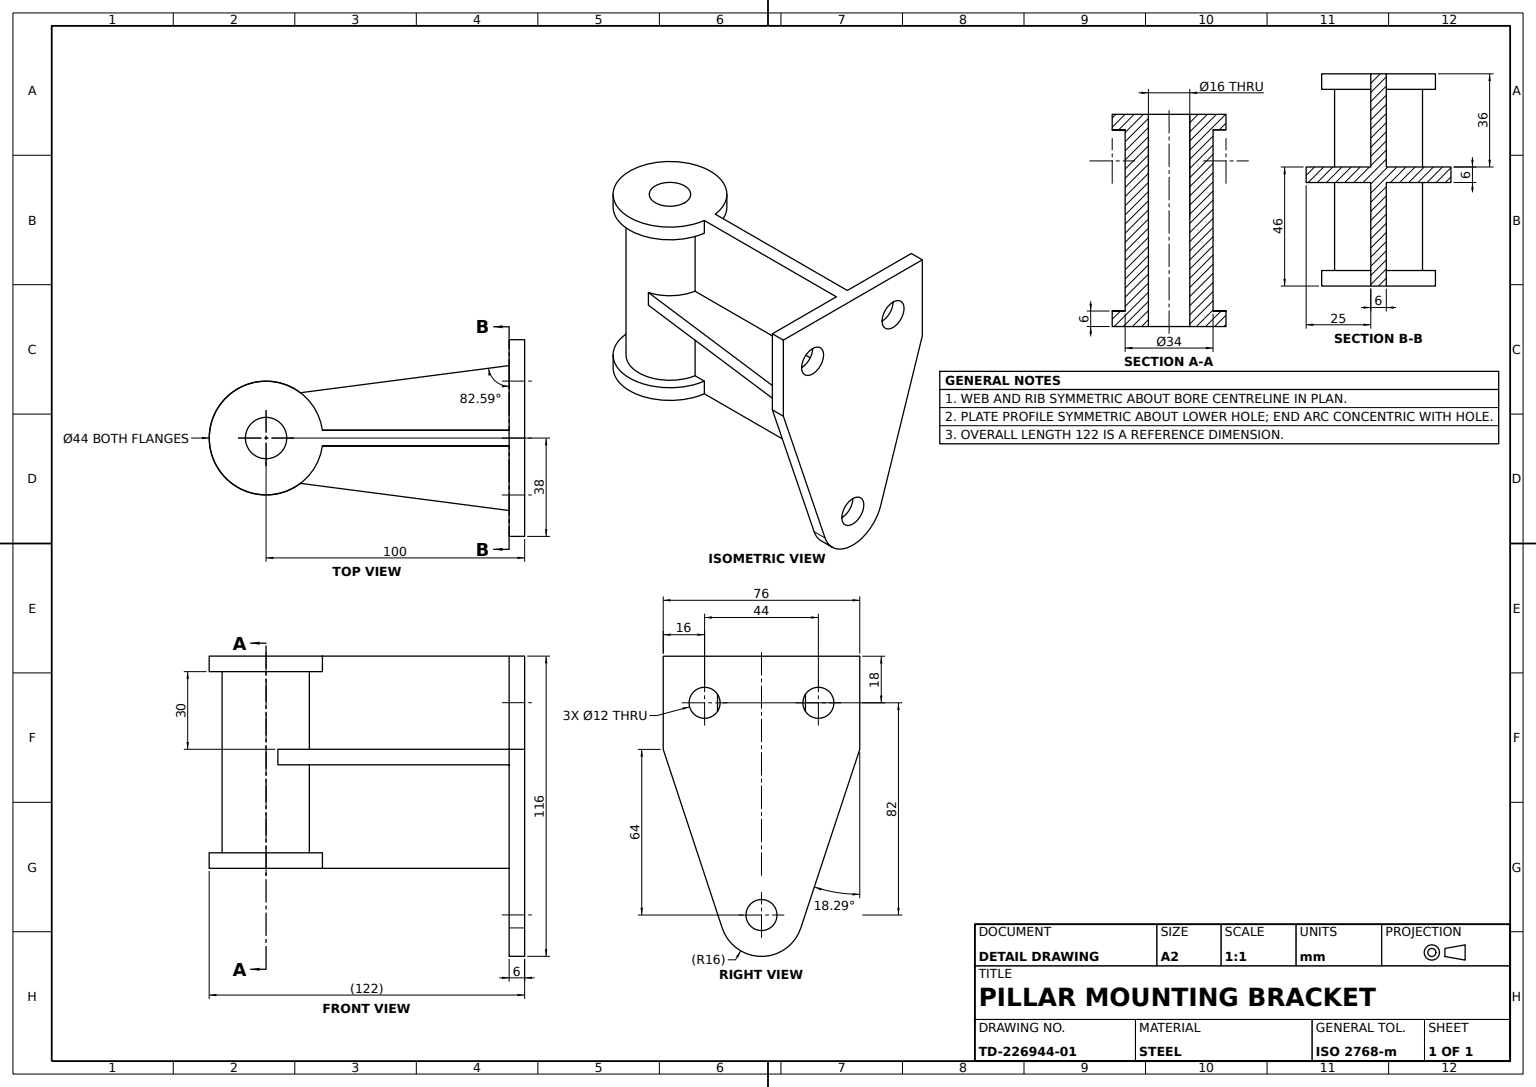
ISO-10303-21;
HEADER;
FILE_DESCRIPTION((''),'2;1');
FILE_NAME('','',(''),(''),'','','');
FILE_SCHEMA(('AUTOMOTIVE_DESIGN'));
ENDSEC;
DATA;
#1=APPLICATION_CONTEXT('');
#2=PRODUCT_CONTEXT('',#1,'mechanical');
#3=PRODUCT('','','',(#2));
#4=PRODUCT_DEFINITION_FORMATION('','',#3);
#5=PRODUCT_DEFINITION_CONTEXT('',#1,'design');
#6=PRODUCT_DEFINITION('','',#4,#5);
#7=PRODUCT_DEFINITION_SHAPE('','',#6);
#8=(LENGTH_UNIT()NAMED_UNIT(*)SI_UNIT(.MILLI.,.METRE.));
#9=(NAMED_UNIT(*)PLANE_ANGLE_UNIT()SI_UNIT($,.RADIAN.));
#10=(NAMED_UNIT(*)SI_UNIT($,.STERADIAN.)SOLID_ANGLE_UNIT());
#11=UNCERTAINTY_MEASURE_WITH_UNIT(LENGTH_MEASURE(0.005),#8,'distance_accuracy_value','');
#12=(GEOMETRIC_REPRESENTATION_CONTEXT(3)GLOBAL_UNCERTAINTY_ASSIGNED_CONTEXT((#11))GLOBAL_UNIT_ASSIGNED_CONTEXT((#8,#9,#10))REPRESENTATION_CONTEXT('',''));
#13=CARTESIAN_POINT('',(83.266799,-3.,-6.));
#14=VERTEX_POINT('',#13);
#15=CARTESIAN_POINT('',(6.,-3.,-6.));
#16=VERTEX_POINT('',#15);
#17=CARTESIAN_POINT('',(106.,-3.,-6.));
#18=DIRECTION('',(-1.,0.,0.));
#19=VECTOR('',#18,1000.);
#20=LINE('',#17,#19);
#21=EDGE_CURVE('',#14,#16,#20,.T.);
#22=ORIENTED_EDGE('',*,*,#21,.T.);
#23=CARTESIAN_POINT('',(6.,-3.,-46.));
#24=VERTEX_POINT('',#23);
#25=CARTESIAN_POINT('',(6.,-3.,36.));
#26=DIRECTION('',(0.,0.,-1.));
#27=VECTOR('',#26,1000.);
#28=LINE('',#25,#27);
#29=EDGE_CURVE('',#16,#24,#28,.T.);
#30=ORIENTED_EDGE('',*,*,#29,.T.);
#31=CARTESIAN_POINT('',(78.205505,-3.,-46.));
#32=VERTEX_POINT('',#31);
#33=DIRECTION('',(1.,0.,0.));
#34=VECTOR('',#33,1000.);
#35=LINE('',#23,#34);
#36=EDGE_CURVE('',#24,#32,#35,.T.);
#37=ORIENTED_EDGE('',*,*,#36,.T.);
#38=CARTESIAN_POINT('',(78.205505,-3.,-40.));
#39=VERTEX_POINT('',#38);
#40=LINE('',#38,#27);
#41=EDGE_CURVE('',#39,#32,#40,.T.);
#42=ORIENTED_EDGE('',*,*,#41,.F.);
#43=CARTESIAN_POINT('',(83.266799,-3.,-40.));
#44=VERTEX_POINT('',#43);
#45=CARTESIAN_POINT('',(0.,-3.,-40.));
#46=LINE('',#45,#19);
#47=EDGE_CURVE('',#39,#44,#46,.F.);
#48=ORIENTED_EDGE('',*,*,#47,.T.);
#49=CARTESIAN_POINT('',(83.266799,-3.,36.));
#50=LINE('',#49,#27);
#51=EDGE_CURVE('',#44,#14,#50,.F.);
#52=ORIENTED_EDGE('',*,*,#51,.T.);
#53=EDGE_LOOP('',(#22,#30,#37,#42,#48,#52));
#54=FACE_BOUND('',#53,.T.);
#55=CARTESIAN_POINT('',(0.,-3.,0.));
#56=DIRECTION('',(0.,-1.,0.));
#57=AXIS2_PLACEMENT_3D('',#55,#56,#26);
#58=PLANE('',#57);
#59=ADVANCED_FACE('',(#54),#58,.T.);
#60=CARTESIAN_POINT('',(83.266799,-3.,0.));
#61=VERTEX_POINT('',#60);
#62=CARTESIAN_POINT('',(83.266799,-3.,30.));
#63=VERTEX_POINT('',#62);
#64=EDGE_CURVE('',#61,#63,#50,.F.);
#65=ORIENTED_EDGE('',*,*,#64,.T.);
#66=CARTESIAN_POINT('',(78.205505,-3.,30.));
#67=VERTEX_POINT('',#66);
#68=CARTESIAN_POINT('',(0.,-3.,30.));
#69=LINE('',#68,#19);
#70=EDGE_CURVE('',#67,#63,#69,.F.);
#71=ORIENTED_EDGE('',*,*,#70,.F.);
#72=CARTESIAN_POINT('',(78.205505,-3.,36.));
#73=VERTEX_POINT('',#72);
#74=LINE('',#72,#27);
#75=EDGE_CURVE('',#73,#67,#74,.T.);
#76=ORIENTED_EDGE('',*,*,#75,.F.);
#77=VERTEX_POINT('',#25);
#78=CARTESIAN_POINT('',(106.,-3.,36.));
#79=LINE('',#78,#19);
#80=EDGE_CURVE('',#73,#77,#79,.T.);
#81=ORIENTED_EDGE('',*,*,#80,.T.);
#82=CARTESIAN_POINT('',(6.,-3.,0.));
#83=VERTEX_POINT('',#82);
#84=EDGE_CURVE('',#77,#83,#28,.T.);
#85=ORIENTED_EDGE('',*,*,#84,.T.);
#86=CARTESIAN_POINT('',(106.,-3.,0.));
#87=LINE('',#86,#19);
#88=EDGE_CURVE('',#61,#83,#87,.T.);
#89=ORIENTED_EDGE('',*,*,#88,.F.);
#90=EDGE_LOOP('',(#65,#71,#76,#81,#85,#89));
#91=FACE_BOUND('',#90,.T.);
#92=ADVANCED_FACE('',(#91),#58,.T.);
#93=CARTESIAN_POINT('',(108.,0.,-46.));
#94=VERTEX_POINT('',#93);
#95=CARTESIAN_POINT('',(100.,0.,-46.));
#96=DIRECTION('',(0.,0.,1.));
#97=AXIS2_PLACEMENT_3D('',#95,#96,#33);
#98=CIRCLE('',#97,8.);
#99=EDGE_CURVE('',#94,#94,#98,.T.);
#100=ORIENTED_EDGE('',*,*,#99,.T.);
#101=EDGE_LOOP('',(#100));
#102=FACE_BOUND('',#101,.T.);
#103=CARTESIAN_POINT('',(6.,3.,-46.));
#104=VERTEX_POINT('',#103);
#105=DIRECTION('',(0.,1.,0.));
#106=VECTOR('',#105,1000.);
#107=LINE('',#23,#106);
#108=EDGE_CURVE('',#24,#104,#107,.T.);
#109=ORIENTED_EDGE('',*,*,#108,.T.);
#110=CARTESIAN_POINT('',(78.205505,3.,-46.));
#111=VERTEX_POINT('',#110);
#112=LINE('',#103,#34);
#113=EDGE_CURVE('',#104,#111,#112,.T.);
#114=ORIENTED_EDGE('',*,*,#113,.T.);
#115=CIRCLE('',#97,22.);
#116=EDGE_CURVE('',#111,#32,#115,.F.);
#117=ORIENTED_EDGE('',*,*,#116,.T.);
#118=ORIENTED_EDGE('',*,*,#36,.F.);
#119=EDGE_LOOP('',(#109,#114,#117,#118));
#120=FACE_BOUND('',#119,.T.);
#121=AXIS2_PLACEMENT_3D('',#23,#96,#33);
#122=PLANE('',#121);
#123=ADVANCED_FACE('',(#102,#120),#122,.F.);
#124=CARTESIAN_POINT('',(83.266799,3.,-6.));
#125=VERTEX_POINT('',#124);
#126=CARTESIAN_POINT('',(6.,3.,-6.));
#127=VERTEX_POINT('',#126);
#128=CARTESIAN_POINT('',(106.,3.,-6.));
#129=LINE('',#128,#19);
#130=EDGE_CURVE('',#125,#127,#129,.T.);
#131=ORIENTED_EDGE('',*,*,#130,.F.);
#132=CARTESIAN_POINT('',(83.266799,3.,-40.));
#133=VERTEX_POINT('',#132);
#134=CARTESIAN_POINT('',(83.266799,3.,36.));
#135=LINE('',#134,#27);
#136=EDGE_CURVE('',#133,#125,#135,.F.);
#137=ORIENTED_EDGE('',*,*,#136,.F.);
#138=CARTESIAN_POINT('',(78.205505,3.,-40.));
#139=VERTEX_POINT('',#138);
#140=CARTESIAN_POINT('',(0.,3.,-40.));
#141=LINE('',#140,#19);
#142=EDGE_CURVE('',#139,#133,#141,.F.);
#143=ORIENTED_EDGE('',*,*,#142,.F.);
#144=LINE('',#138,#27);
#145=EDGE_CURVE('',#139,#111,#144,.T.);
#146=ORIENTED_EDGE('',*,*,#145,.T.);
#147=ORIENTED_EDGE('',*,*,#113,.F.);
#148=CARTESIAN_POINT('',(6.,3.,36.));
#149=LINE('',#148,#27);
#150=EDGE_CURVE('',#127,#104,#149,.T.);
#151=ORIENTED_EDGE('',*,*,#150,.F.);
#152=EDGE_LOOP('',(#131,#137,#143,#146,#147,#151));
#153=FACE_BOUND('',#152,.T.);
#154=CARTESIAN_POINT('',(0.,3.,0.));
#155=AXIS2_PLACEMENT_3D('',#154,#56,#26);
#156=PLANE('',#155);
#157=ADVANCED_FACE('',(#153),#156,.F.);
#158=ORIENTED_EDGE('',*,*,#80,.F.);
#159=CARTESIAN_POINT('',(78.205505,3.,36.));
#160=VERTEX_POINT('',#159);
#161=CARTESIAN_POINT('',(100.,0.,36.));
#162=AXIS2_PLACEMENT_3D('',#161,#96,#33);
#163=CIRCLE('',#162,22.);
#164=EDGE_CURVE('',#160,#73,#163,.F.);
#165=ORIENTED_EDGE('',*,*,#164,.F.);
#166=VERTEX_POINT('',#148);
#167=CARTESIAN_POINT('',(106.,3.,36.));
#168=LINE('',#167,#19);
#169=EDGE_CURVE('',#160,#166,#168,.T.);
#170=ORIENTED_EDGE('',*,*,#169,.T.);
#171=CARTESIAN_POINT('',(6.,38.,36.));
#172=VERTEX_POINT('',#171);
#173=CARTESIAN_POINT('',(6.,-38.,36.));
#174=LINE('',#173,#106);
#175=EDGE_CURVE('',#166,#172,#174,.T.);
#176=ORIENTED_EDGE('',*,*,#175,.T.);
#177=CARTESIAN_POINT('',(0.,38.,36.));
#178=VERTEX_POINT('',#177);
#179=LINE('',#171,#19);
#180=EDGE_CURVE('',#172,#178,#179,.T.);
#181=ORIENTED_EDGE('',*,*,#180,.T.);
#182=CARTESIAN_POINT('',(0.,-38.,36.));
#183=VERTEX_POINT('',#182);
#184=LINE('',#182,#106);
#185=EDGE_CURVE('',#183,#178,#184,.T.);
#186=ORIENTED_EDGE('',*,*,#185,.F.);
#187=VERTEX_POINT('',#173);
#188=LINE('',#173,#19);
#189=EDGE_CURVE('',#187,#183,#188,.T.);
#190=ORIENTED_EDGE('',*,*,#189,.F.);
#191=EDGE_CURVE('',#187,#77,#174,.T.);
#192=ORIENTED_EDGE('',*,*,#191,.T.);
#193=EDGE_LOOP('',(#158,#165,#170,#176,#181,#186,#190,#192));
#194=FACE_BOUND('',#193,.T.);
#195=CARTESIAN_POINT('',(92.,0.,36.));
#196=VERTEX_POINT('',#195);
#197=AXIS2_PLACEMENT_3D('',#161,#26,#18);
#198=CIRCLE('',#197,8.);
#199=EDGE_CURVE('',#196,#196,#198,.T.);
#200=ORIENTED_EDGE('',*,*,#199,.T.);
#201=EDGE_LOOP('',(#200));
#202=FACE_BOUND('',#201,.T.);
#203=AXIS2_PLACEMENT_3D('',#173,#96,#33);
#204=PLANE('',#203);
#205=ADVANCED_FACE('',(#194,#202),#204,.T.);
#206=ORIENTED_EDGE('',*,*,#130,.T.);
#207=CARTESIAN_POINT('',(6.,28.,-6.));
#208=VERTEX_POINT('',#207);
#209=LINE('',#126,#106);
#210=EDGE_CURVE('',#127,#208,#209,.T.);
#211=ORIENTED_EDGE('',*,*,#210,.T.);
#212=CARTESIAN_POINT('',(95.429705,16.374138,-6.));
#213=VERTEX_POINT('',#212);
#214=DIRECTION('',(0.991655617,-0.12891523,0.));
#215=VECTOR('',#214,1000.);
#216=LINE('',#207,#215);
#217=EDGE_CURVE('',#208,#213,#216,.T.);
#218=ORIENTED_EDGE('',*,*,#217,.T.);
#219=CARTESIAN_POINT('',(100.,0.,-6.));
#220=AXIS2_PLACEMENT_3D('',#219,#26,#18);
#221=CIRCLE('',#220,17.);
#222=EDGE_CURVE('',#125,#213,#221,.T.);
#223=ORIENTED_EDGE('',*,*,#222,.F.);
#224=EDGE_LOOP('',(#206,#211,#218,#223));
#225=FACE_BOUND('',#224,.T.);
#226=CARTESIAN_POINT('',(0.,0.,-6.));
#227=AXIS2_PLACEMENT_3D('',#226,#26,#18);
#228=PLANE('',#227);
#229=ADVANCED_FACE('',(#225),#228,.T.);
#230=ORIENTED_EDGE('',*,*,#199,.F.);
#231=EDGE_LOOP('',(#230));
#232=FACE_BOUND('',#231,.T.);
#233=ORIENTED_EDGE('',*,*,#99,.F.);
#234=EDGE_LOOP('',(#233));
#235=FACE_BOUND('',#234,.T.);
#236=CYLINDRICAL_SURFACE('',#197,8.);
#237=ADVANCED_FACE('',(#232,#235),#236,.F.);
#238=CARTESIAN_POINT('',(6.,-28.,0.));
#239=VERTEX_POINT('',#238);
#240=CARTESIAN_POINT('',(95.429705,-16.374138,0.));
#241=VERTEX_POINT('',#240);
#242=DIRECTION('',(0.991655617,0.12891523,0.));
#243=VECTOR('',#242,1000.);
#244=LINE('',#238,#243);
#245=EDGE_CURVE('',#239,#241,#244,.T.);
#246=ORIENTED_EDGE('',*,*,#245,.T.);
#247=CARTESIAN_POINT('',(100.,0.,0.));
#248=AXIS2_PLACEMENT_3D('',#247,#96,#33);
#249=CIRCLE('',#248,17.);
#250=EDGE_CURVE('',#61,#241,#249,.T.);
#251=ORIENTED_EDGE('',*,*,#250,.F.);
#252=ORIENTED_EDGE('',*,*,#88,.T.);
#253=VECTOR('',#56,1000.);
#254=LINE('',#82,#253);
#255=EDGE_CURVE('',#83,#239,#254,.T.);
#256=ORIENTED_EDGE('',*,*,#255,.T.);
#257=EDGE_LOOP('',(#246,#251,#252,#256));
#258=FACE_BOUND('',#257,.T.);
#259=CARTESIAN_POINT('',(0.,0.,0.));
#260=AXIS2_PLACEMENT_3D('',#259,#96,#33);
#261=PLANE('',#260);
#262=ADVANCED_FACE('',(#258),#261,.T.);
#263=CARTESIAN_POINT('',(6.,-22.,24.));
#264=VERTEX_POINT('',#263);
#265=CARTESIAN_POINT('',(6.,-22.,18.));
#266=AXIS2_PLACEMENT_3D('',#265,#18,#96);
#267=CIRCLE('',#266,6.);
#268=EDGE_CURVE('',#264,#264,#267,.T.);
#269=ORIENTED_EDGE('',*,*,#268,.F.);
#270=EDGE_LOOP('',(#269));
#271=FACE_BOUND('',#270,.T.);
#272=CARTESIAN_POINT('',(0.,-22.,24.));
#273=VERTEX_POINT('',#272);
#274=CARTESIAN_POINT('',(0.,-22.,18.));
#275=AXIS2_PLACEMENT_3D('',#274,#18,#96);
#276=CIRCLE('',#275,6.);
#277=EDGE_CURVE('',#273,#273,#276,.T.);
#278=ORIENTED_EDGE('',*,*,#277,.T.);
#279=EDGE_LOOP('',(#278));
#280=FACE_BOUND('',#279,.T.);
#281=CYLINDRICAL_SURFACE('',#266,6.);
#282=ADVANCED_FACE('',(#271,#280),#281,.F.);
#283=CARTESIAN_POINT('',(95.429705,-16.374138,-6.));
#284=VERTEX_POINT('',#283);
#285=AXIS2_PLACEMENT_3D('',#219,#96,#33);
#286=CIRCLE('',#285,17.);
#287=EDGE_CURVE('',#14,#284,#286,.T.);
#288=ORIENTED_EDGE('',*,*,#287,.T.);
#289=CARTESIAN_POINT('',(6.,-28.,-6.));
#290=VERTEX_POINT('',#289);
#291=LINE('',#289,#243);
#292=EDGE_CURVE('',#290,#284,#291,.T.);
#293=ORIENTED_EDGE('',*,*,#292,.F.);
#294=LINE('',#15,#253);
#295=EDGE_CURVE('',#16,#290,#294,.T.);
#296=ORIENTED_EDGE('',*,*,#295,.F.);
#297=ORIENTED_EDGE('',*,*,#21,.F.);
#298=EDGE_LOOP('',(#288,#293,#296,#297));
#299=FACE_BOUND('',#298,.T.);
#300=AXIS2_PLACEMENT_3D('',#226,#96,#33);
#301=PLANE('',#300);
#302=ADVANCED_FACE('',(#299),#301,.F.);
#303=CARTESIAN_POINT('',(95.429705,16.374138,0.));
#304=VERTEX_POINT('',#303);
#305=CARTESIAN_POINT('',(95.429705,16.374138,36.));
#306=LINE('',#305,#27);
#307=EDGE_CURVE('',#304,#213,#306,.T.);
#308=ORIENTED_EDGE('',*,*,#307,.F.);
#309=CARTESIAN_POINT('',(83.266799,3.,0.));
#310=VERTEX_POINT('',#309);
#311=AXIS2_PLACEMENT_3D('',#247,#26,#18);
#312=CIRCLE('',#311,17.);
#313=EDGE_CURVE('',#310,#304,#312,.T.);
#314=ORIENTED_EDGE('',*,*,#313,.F.);
#315=CARTESIAN_POINT('',(83.266799,3.,30.));
#316=VERTEX_POINT('',#315);
#317=EDGE_CURVE('',#310,#316,#135,.F.);
#318=ORIENTED_EDGE('',*,*,#317,.T.);
#319=CARTESIAN_POINT('',(100.,0.,30.));
#320=AXIS2_PLACEMENT_3D('',#319,#96,#33);
#321=CIRCLE('',#320,17.);
#322=EDGE_CURVE('',#316,#63,#321,.F.);
#323=ORIENTED_EDGE('',*,*,#322,.T.);
#324=ORIENTED_EDGE('',*,*,#64,.F.);
#325=ORIENTED_EDGE('',*,*,#250,.T.);
#326=CARTESIAN_POINT('',(95.429705,-16.374138,36.));
#327=LINE('',#326,#27);
#328=EDGE_CURVE('',#241,#284,#327,.T.);
#329=ORIENTED_EDGE('',*,*,#328,.T.);
#330=ORIENTED_EDGE('',*,*,#287,.F.);
#331=ORIENTED_EDGE('',*,*,#51,.F.);
#332=CARTESIAN_POINT('',(100.,0.,-40.));
#333=AXIS2_PLACEMENT_3D('',#332,#96,#33);
#334=CIRCLE('',#333,17.);
#335=EDGE_CURVE('',#133,#44,#334,.F.);
#336=ORIENTED_EDGE('',*,*,#335,.F.);
#337=ORIENTED_EDGE('',*,*,#136,.T.);
#338=ORIENTED_EDGE('',*,*,#222,.T.);
#339=EDGE_LOOP('',(#308,#314,#318,#323,#324,#325,#329,#330,#331,#336,#337,#338));
#340=FACE_BOUND('',#339,.T.);
#341=CYLINDRICAL_SURFACE('',#197,17.);
#342=ADVANCED_FACE('',(#340),#341,.T.);
#343=ORIENTED_EDGE('',*,*,#307,.T.);
#344=ORIENTED_EDGE('',*,*,#217,.F.);
#345=CARTESIAN_POINT('',(6.,28.,0.));
#346=VERTEX_POINT('',#345);
#347=VECTOR('',#96,1000.);
#348=LINE('',#207,#347);
#349=EDGE_CURVE('',#208,#346,#348,.T.);
#350=ORIENTED_EDGE('',*,*,#349,.T.);
#351=LINE('',#345,#215);
#352=EDGE_CURVE('',#346,#304,#351,.T.);
#353=ORIENTED_EDGE('',*,*,#352,.T.);
#354=EDGE_LOOP('',(#343,#344,#350,#353));
#355=FACE_BOUND('',#354,.T.);
#356=DIRECTION('',(-0.12891523,-0.991655617,0.));
#357=AXIS2_PLACEMENT_3D('',#207,#356,#214);
#358=PLANE('',#357);
#359=ADVANCED_FACE('',(#355),#358,.F.);
#360=CARTESIAN_POINT('',(6.,-15.192006,-69.020254));
#361=VERTEX_POINT('',#360);
#362=CARTESIAN_POINT('',(0.,-15.192006,-69.020254));
#363=VERTEX_POINT('',#362);
#364=LINE('',#360,#19);
#365=EDGE_CURVE('',#361,#363,#364,.T.);
#366=ORIENTED_EDGE('',*,*,#365,.F.);
#367=CARTESIAN_POINT('',(6.,-38.,0.));
#368=VERTEX_POINT('',#367);
#369=DIRECTION('',(0.,-0.313765856,0.949500389));
#370=VECTOR('',#369,1000.);
#371=LINE('',#360,#370);
#372=EDGE_CURVE('',#361,#368,#371,.T.);
#373=ORIENTED_EDGE('',*,*,#372,.T.);
#374=CARTESIAN_POINT('',(0.,-38.,0.));
#375=VERTEX_POINT('',#374);
#376=LINE('',#367,#19);
#377=EDGE_CURVE('',#368,#375,#376,.T.);
#378=ORIENTED_EDGE('',*,*,#377,.T.);
#379=LINE('',#362,#370);
#380=EDGE_CURVE('',#363,#375,#379,.T.);
#381=ORIENTED_EDGE('',*,*,#380,.F.);
#382=EDGE_LOOP('',(#366,#373,#378,#381));
#383=FACE_BOUND('',#382,.T.);
#384=DIRECTION('',(0.,-0.949500389,-0.313765856));
#385=DIRECTION('',(0.,0.313765856,-0.949500389));
#386=AXIS2_PLACEMENT_3D('',#360,#384,#385);
#387=PLANE('',#386);
#388=ADVANCED_FACE('',(#383),#387,.T.);
#389=ORIENTED_EDGE('',*,*,#164,.T.);
#390=ORIENTED_EDGE('',*,*,#75,.T.);
#391=CARTESIAN_POINT('',(78.205505,3.,30.));
#392=VERTEX_POINT('',#391);
#393=CIRCLE('',#320,22.);
#394=EDGE_CURVE('',#392,#67,#393,.F.);
#395=ORIENTED_EDGE('',*,*,#394,.F.);
#396=LINE('',#159,#27);
#397=EDGE_CURVE('',#160,#392,#396,.T.);
#398=ORIENTED_EDGE('',*,*,#397,.F.);
#399=EDGE_LOOP('',(#389,#390,#395,#398));
#400=FACE_BOUND('',#399,.T.);
#401=CYLINDRICAL_SURFACE('',#197,22.);
#402=ADVANCED_FACE('',(#400),#401,.T.);
#403=ORIENTED_EDGE('',*,*,#47,.F.);
#404=CIRCLE('',#333,22.);
#405=EDGE_CURVE('',#139,#39,#404,.F.);
#406=ORIENTED_EDGE('',*,*,#405,.F.);
#407=ORIENTED_EDGE('',*,*,#142,.T.);
#408=ORIENTED_EDGE('',*,*,#335,.T.);
#409=EDGE_LOOP('',(#403,#406,#407,#408));
#410=FACE_BOUND('',#409,.T.);
#411=PLANE('',#333);
#412=ADVANCED_FACE('',(#410),#411,.T.);
#413=ORIENTED_EDGE('',*,*,#322,.F.);
#414=CARTESIAN_POINT('',(0.,3.,30.));
#415=LINE('',#414,#19);
#416=EDGE_CURVE('',#392,#316,#415,.F.);
#417=ORIENTED_EDGE('',*,*,#416,.F.);
#418=ORIENTED_EDGE('',*,*,#394,.T.);
#419=ORIENTED_EDGE('',*,*,#70,.T.);
#420=EDGE_LOOP('',(#413,#417,#418,#419));
#421=FACE_BOUND('',#420,.T.);
#422=PLANE('',#320);
#423=ADVANCED_FACE('',(#421),#422,.F.);
#424=CARTESIAN_POINT('',(6.,22.,24.));
#425=VERTEX_POINT('',#424);
#426=CARTESIAN_POINT('',(6.,22.,18.));
#427=AXIS2_PLACEMENT_3D('',#426,#18,#96);
#428=CIRCLE('',#427,6.);
#429=EDGE_CURVE('',#425,#425,#428,.T.);
#430=ORIENTED_EDGE('',*,*,#429,.F.);
#431=EDGE_LOOP('',(#430));
#432=FACE_BOUND('',#431,.T.);
#433=CARTESIAN_POINT('',(0.,22.,24.));
#434=VERTEX_POINT('',#433);
#435=CARTESIAN_POINT('',(0.,22.,18.));
#436=AXIS2_PLACEMENT_3D('',#435,#18,#96);
#437=CIRCLE('',#436,6.);
#438=EDGE_CURVE('',#434,#434,#437,.T.);
#439=ORIENTED_EDGE('',*,*,#438,.T.);
#440=EDGE_LOOP('',(#439));
#441=FACE_BOUND('',#440,.T.);
#442=CYLINDRICAL_SURFACE('',#427,6.);
#443=ADVANCED_FACE('',(#432,#441),#442,.F.);
#444=ORIENTED_EDGE('',*,*,#169,.F.);
#445=ORIENTED_EDGE('',*,*,#397,.T.);
#446=ORIENTED_EDGE('',*,*,#416,.T.);
#447=ORIENTED_EDGE('',*,*,#317,.F.);
#448=CARTESIAN_POINT('',(6.,3.,0.));
#449=VERTEX_POINT('',#448);
#450=CARTESIAN_POINT('',(106.,3.,0.));
#451=LINE('',#450,#19);
#452=EDGE_CURVE('',#310,#449,#451,.T.);
#453=ORIENTED_EDGE('',*,*,#452,.T.);
#454=EDGE_CURVE('',#166,#449,#149,.T.);
#455=ORIENTED_EDGE('',*,*,#454,.F.);
#456=EDGE_LOOP('',(#444,#445,#446,#447,#453,#455));
#457=FACE_BOUND('',#456,.T.);
#458=ADVANCED_FACE('',(#457),#156,.F.);
#459=CARTESIAN_POINT('',(6.,38.,0.));
#460=VERTEX_POINT('',#459);
#461=CARTESIAN_POINT('',(6.,15.192006,-69.020254));
#462=VERTEX_POINT('',#461);
#463=DIRECTION('',(0.,-0.313765856,-0.949500389));
#464=VECTOR('',#463,1000.);
#465=LINE('',#459,#464);
#466=EDGE_CURVE('',#460,#462,#465,.T.);
#467=ORIENTED_EDGE('',*,*,#466,.T.);
#468=CARTESIAN_POINT('',(0.,15.192006,-69.020254));
#469=VERTEX_POINT('',#468);
#470=LINE('',#461,#19);
#471=EDGE_CURVE('',#462,#469,#470,.T.);
#472=ORIENTED_EDGE('',*,*,#471,.T.);
#473=CARTESIAN_POINT('',(0.,38.,0.));
#474=VERTEX_POINT('',#473);
#475=LINE('',#473,#464);
#476=EDGE_CURVE('',#474,#469,#475,.T.);
#477=ORIENTED_EDGE('',*,*,#476,.F.);
#478=LINE('',#459,#19);
#479=EDGE_CURVE('',#460,#474,#478,.T.);
#480=ORIENTED_EDGE('',*,*,#479,.F.);
#481=EDGE_LOOP('',(#467,#472,#477,#480));
#482=FACE_BOUND('',#481,.T.);
#483=DIRECTION('',(0.,0.949500389,-0.313765856));
#484=DIRECTION('',(0.,0.313765856,0.949500389));
#485=AXIS2_PLACEMENT_3D('',#459,#483,#484);
#486=PLANE('',#485);
#487=ADVANCED_FACE('',(#482),#486,.T.);
#488=ORIENTED_EDGE('',*,*,#429,.T.);
#489=EDGE_LOOP('',(#488));
#490=FACE_BOUND('',#489,.T.);
#491=CARTESIAN_POINT('',(6.,0.,-58.));
#492=VERTEX_POINT('',#491);
#493=CARTESIAN_POINT('',(6.,0.,-64.));
#494=AXIS2_PLACEMENT_3D('',#493,#18,#96);
#495=CIRCLE('',#494,6.);
#496=EDGE_CURVE('',#492,#492,#495,.T.);
#497=ORIENTED_EDGE('',*,*,#496,.T.);
#498=EDGE_LOOP('',(#497));
#499=FACE_BOUND('',#498,.T.);
#500=LINE('',#367,#347);
#501=EDGE_CURVE('',#368,#187,#500,.T.);
#502=ORIENTED_EDGE('',*,*,#501,.F.);
#503=ORIENTED_EDGE('',*,*,#372,.F.);
#504=AXIS2_PLACEMENT_3D('',#493,#18,#105);
#505=CIRCLE('',#504,16.);
#506=EDGE_CURVE('',#462,#361,#505,.T.);
#507=ORIENTED_EDGE('',*,*,#506,.F.);
#508=ORIENTED_EDGE('',*,*,#466,.F.);
#509=LINE('',#171,#27);
#510=EDGE_CURVE('',#172,#460,#509,.T.);
#511=ORIENTED_EDGE('',*,*,#510,.F.);
#512=ORIENTED_EDGE('',*,*,#175,.F.);
#513=ORIENTED_EDGE('',*,*,#454,.T.);
#514=LINE('',#448,#106);
#515=EDGE_CURVE('',#449,#346,#514,.T.);
#516=ORIENTED_EDGE('',*,*,#515,.T.);
#517=ORIENTED_EDGE('',*,*,#349,.F.);
#518=ORIENTED_EDGE('',*,*,#210,.F.);
#519=ORIENTED_EDGE('',*,*,#150,.T.);
#520=ORIENTED_EDGE('',*,*,#108,.F.);
#521=ORIENTED_EDGE('',*,*,#29,.F.);
#522=ORIENTED_EDGE('',*,*,#295,.T.);
#523=LINE('',#289,#347);
#524=EDGE_CURVE('',#290,#239,#523,.T.);
#525=ORIENTED_EDGE('',*,*,#524,.T.);
#526=ORIENTED_EDGE('',*,*,#255,.F.);
#527=ORIENTED_EDGE('',*,*,#84,.F.);
#528=ORIENTED_EDGE('',*,*,#191,.F.);
#529=EDGE_LOOP('',(#502,#503,#507,#508,#511,#512,#513,#516,#517,#518,#519,#520,#521,#522,#525,#526,#527,#528));
#530=FACE_BOUND('',#529,.T.);
#531=ORIENTED_EDGE('',*,*,#268,.T.);
#532=EDGE_LOOP('',(#531));
#533=FACE_BOUND('',#532,.T.);
#534=PLANE('',#494);
#535=ADVANCED_FACE('',(#490,#499,#530,#533),#534,.F.);
#536=LINE('',#177,#27);
#537=EDGE_CURVE('',#178,#474,#536,.T.);
#538=ORIENTED_EDGE('',*,*,#537,.F.);
#539=ORIENTED_EDGE('',*,*,#180,.F.);
#540=ORIENTED_EDGE('',*,*,#510,.T.);
#541=ORIENTED_EDGE('',*,*,#479,.T.);
#542=EDGE_LOOP('',(#538,#539,#540,#541));
#543=FACE_BOUND('',#542,.T.);
#544=AXIS2_PLACEMENT_3D('',#171,#105,#96);
#545=PLANE('',#544);
#546=ADVANCED_FACE('',(#543),#545,.T.);
#547=ORIENTED_EDGE('',*,*,#185,.T.);
#548=ORIENTED_EDGE('',*,*,#537,.T.);
#549=ORIENTED_EDGE('',*,*,#476,.T.);
#550=CARTESIAN_POINT('',(0.,0.,-64.));
#551=AXIS2_PLACEMENT_3D('',#550,#18,#105);
#552=CIRCLE('',#551,16.);
#553=EDGE_CURVE('',#469,#363,#552,.T.);
#554=ORIENTED_EDGE('',*,*,#553,.T.);
#555=ORIENTED_EDGE('',*,*,#380,.T.);
#556=LINE('',#374,#347);
#557=EDGE_CURVE('',#375,#183,#556,.T.);
#558=ORIENTED_EDGE('',*,*,#557,.T.);
#559=EDGE_LOOP('',(#547,#548,#549,#554,#555,#558));
#560=FACE_BOUND('',#559,.T.);
#561=ORIENTED_EDGE('',*,*,#277,.F.);
#562=EDGE_LOOP('',(#561));
#563=FACE_BOUND('',#562,.T.);
#564=ORIENTED_EDGE('',*,*,#438,.F.);
#565=EDGE_LOOP('',(#564));
#566=FACE_BOUND('',#565,.T.);
#567=CARTESIAN_POINT('',(0.,0.,-58.));
#568=VERTEX_POINT('',#567);
#569=AXIS2_PLACEMENT_3D('',#550,#18,#96);
#570=CIRCLE('',#569,6.);
#571=EDGE_CURVE('',#568,#568,#570,.T.);
#572=ORIENTED_EDGE('',*,*,#571,.F.);
#573=EDGE_LOOP('',(#572));
#574=FACE_BOUND('',#573,.T.);
#575=PLANE('',#569);
#576=ADVANCED_FACE('',(#560,#563,#566,#574),#575,.T.);
#577=ORIENTED_EDGE('',*,*,#352,.F.);
#578=ORIENTED_EDGE('',*,*,#515,.F.);
#579=ORIENTED_EDGE('',*,*,#452,.F.);
#580=ORIENTED_EDGE('',*,*,#313,.T.);
#581=EDGE_LOOP('',(#577,#578,#579,#580));
#582=FACE_BOUND('',#581,.T.);
#583=AXIS2_PLACEMENT_3D('',#259,#26,#18);
#584=PLANE('',#583);
#585=ADVANCED_FACE('',(#582),#584,.F.);
#586=ORIENTED_EDGE('',*,*,#496,.F.);
#587=EDGE_LOOP('',(#586));
#588=FACE_BOUND('',#587,.T.);
#589=ORIENTED_EDGE('',*,*,#571,.T.);
#590=EDGE_LOOP('',(#589));
#591=FACE_BOUND('',#590,.T.);
#592=CYLINDRICAL_SURFACE('',#494,6.);
#593=ADVANCED_FACE('',(#588,#591),#592,.F.);
#594=ORIENTED_EDGE('',*,*,#506,.T.);
#595=ORIENTED_EDGE('',*,*,#365,.T.);
#596=ORIENTED_EDGE('',*,*,#553,.F.);
#597=ORIENTED_EDGE('',*,*,#471,.F.);
#598=EDGE_LOOP('',(#594,#595,#596,#597));
#599=FACE_BOUND('',#598,.T.);
#600=CYLINDRICAL_SURFACE('',#494,16.);
#601=ADVANCED_FACE('',(#599),#600,.T.);
#602=ORIENTED_EDGE('',*,*,#377,.F.);
#603=ORIENTED_EDGE('',*,*,#501,.T.);
#604=ORIENTED_EDGE('',*,*,#189,.T.);
#605=ORIENTED_EDGE('',*,*,#557,.F.);
#606=EDGE_LOOP('',(#602,#603,#604,#605));
#607=FACE_BOUND('',#606,.T.);
#608=AXIS2_PLACEMENT_3D('',#367,#56,#26);
#609=PLANE('',#608);
#610=ADVANCED_FACE('',(#607),#609,.T.);
#611=ORIENTED_EDGE('',*,*,#116,.F.);
#612=ORIENTED_EDGE('',*,*,#145,.F.);
#613=ORIENTED_EDGE('',*,*,#405,.T.);
#614=ORIENTED_EDGE('',*,*,#41,.T.);
#615=EDGE_LOOP('',(#611,#612,#613,#614));
#616=FACE_BOUND('',#615,.T.);
#617=AXIS2_PLACEMENT_3D('',#332,#26,#18);
#618=CYLINDRICAL_SURFACE('',#617,22.);
#619=ADVANCED_FACE('',(#616),#618,.T.);
#620=ORIENTED_EDGE('',*,*,#328,.F.);
#621=ORIENTED_EDGE('',*,*,#245,.F.);
#622=ORIENTED_EDGE('',*,*,#524,.F.);
#623=ORIENTED_EDGE('',*,*,#292,.T.);
#624=EDGE_LOOP('',(#620,#621,#622,#623));
#625=FACE_BOUND('',#624,.T.);
#626=DIRECTION('',(0.12891523,-0.991655617,0.));
#627=AXIS2_PLACEMENT_3D('',#289,#626,#242);
#628=PLANE('',#627);
#629=ADVANCED_FACE('',(#625),#628,.T.);
#630=CLOSED_SHELL('',(#59,#92,#123,#157,#205,#229,#237,#262,#282,#302,#342,#359,#388,#402,#412,#423,#443,#458,#487,#535,#546,#576,#585,#593,#601,#610,#619,#629));
#631=MANIFOLD_SOLID_BREP('',#630);
#632=ADVANCED_BREP_SHAPE_REPRESENTATION('',(#631),#12);
#633=SHAPE_DEFINITION_REPRESENTATION(#7,#632);
ENDSEC;
END-ISO-10303-21;
